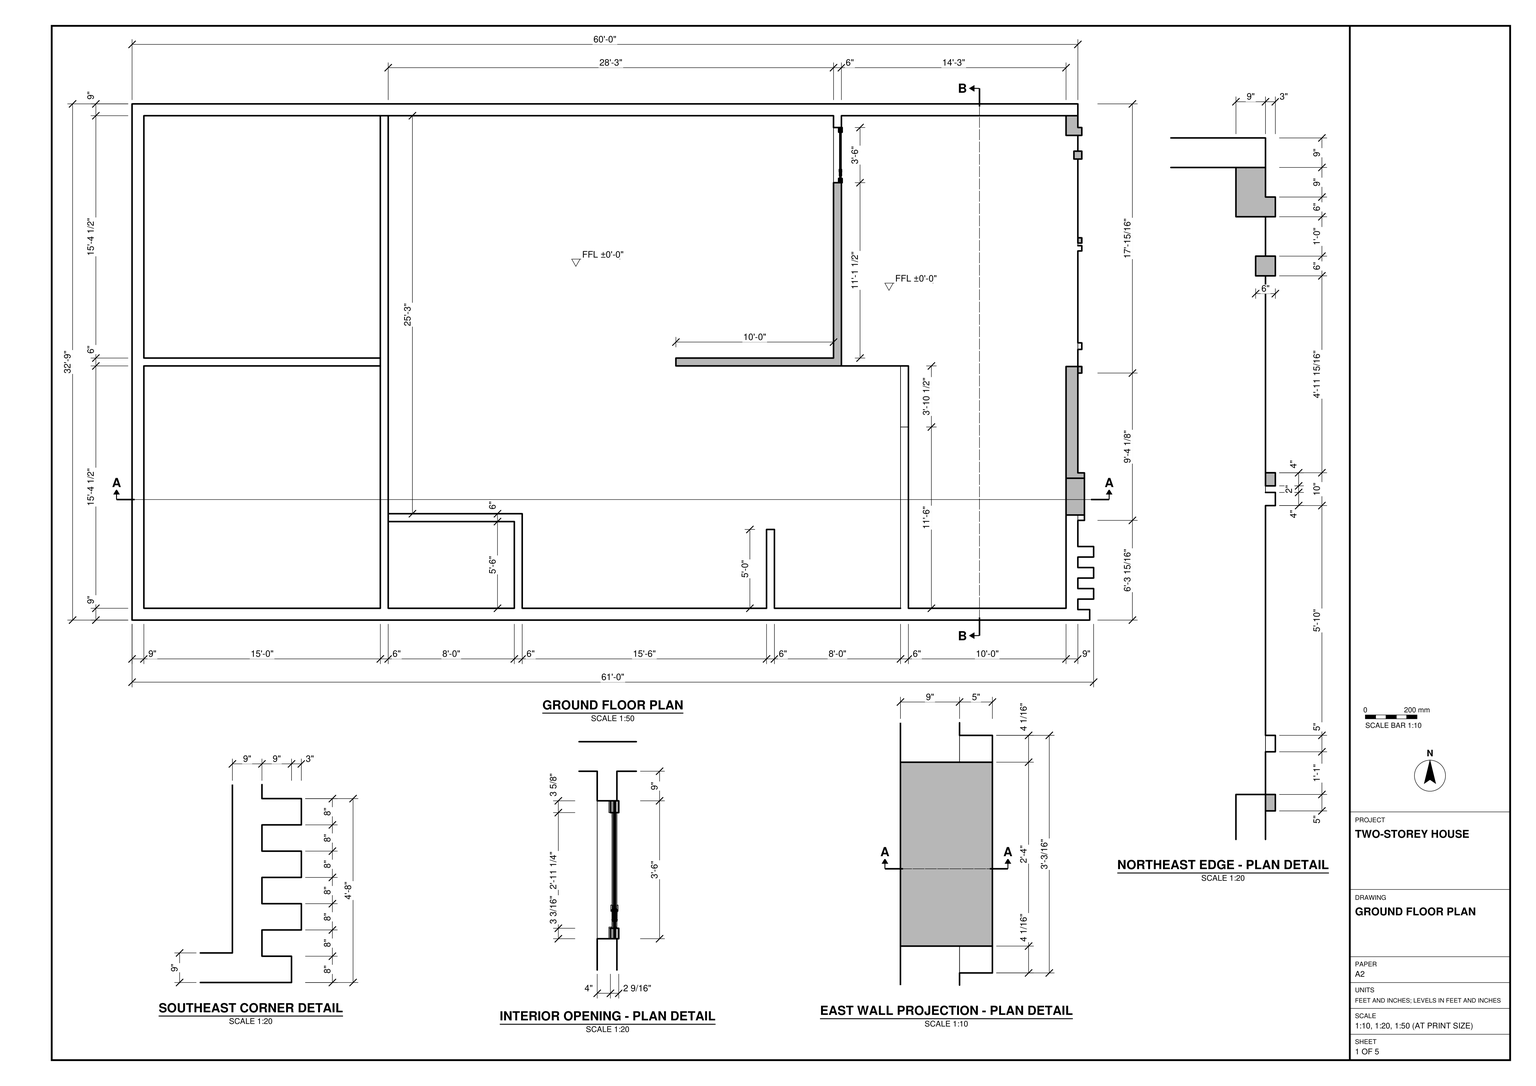
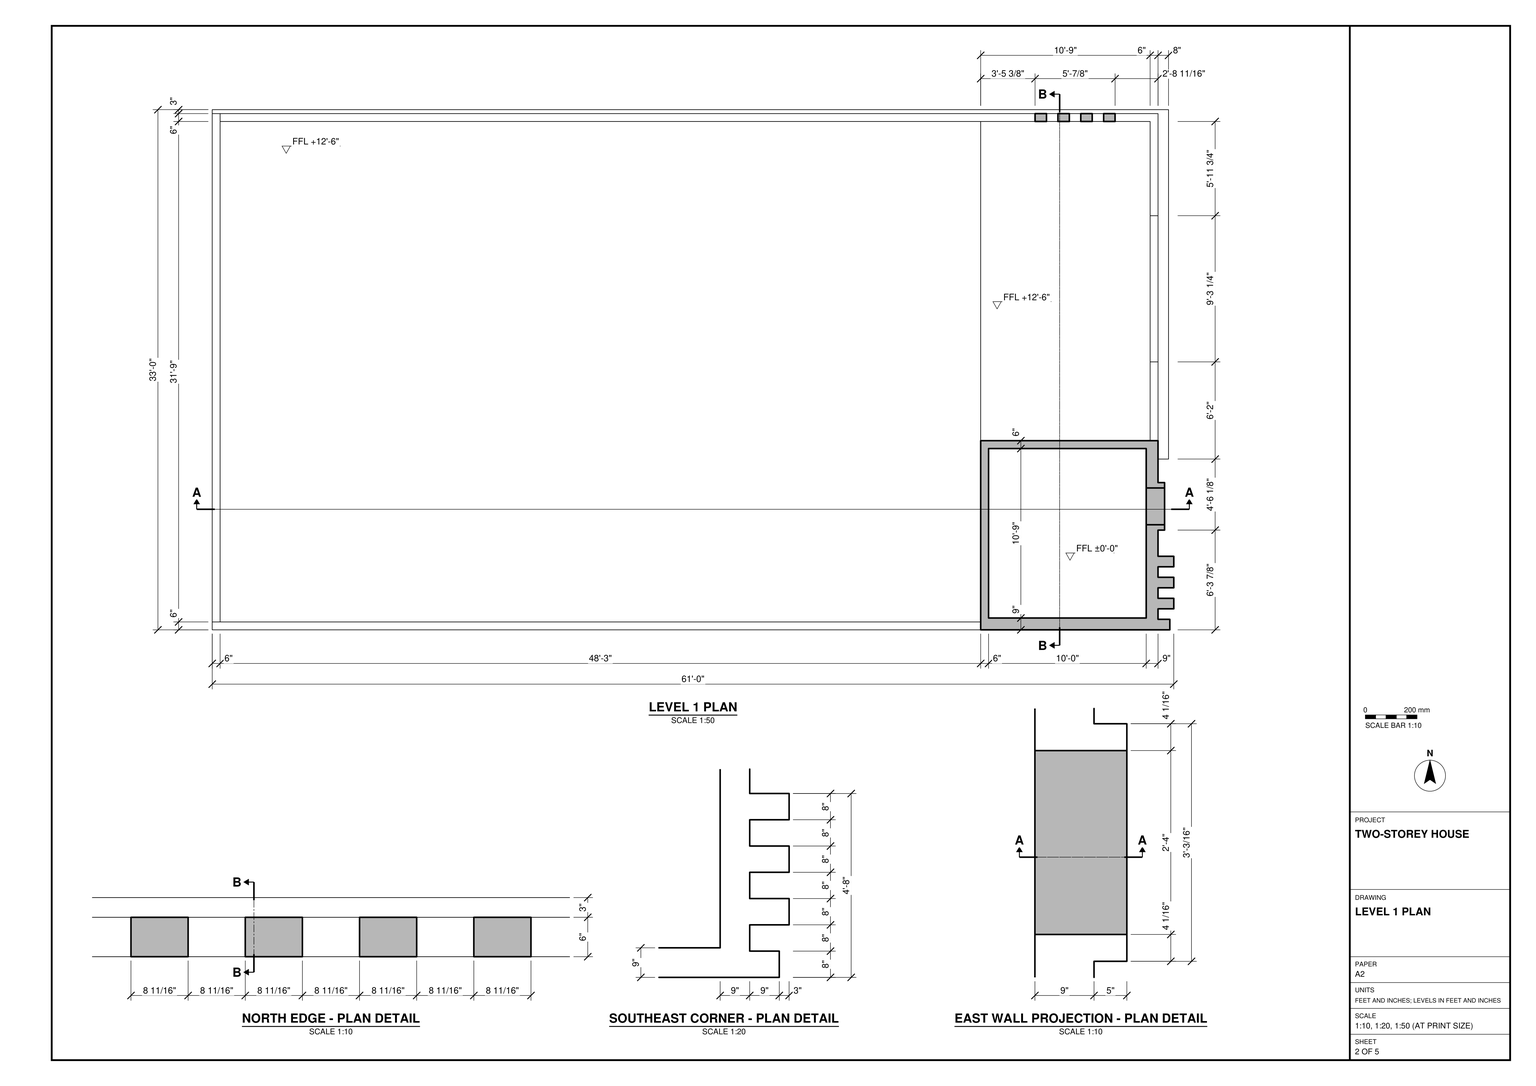
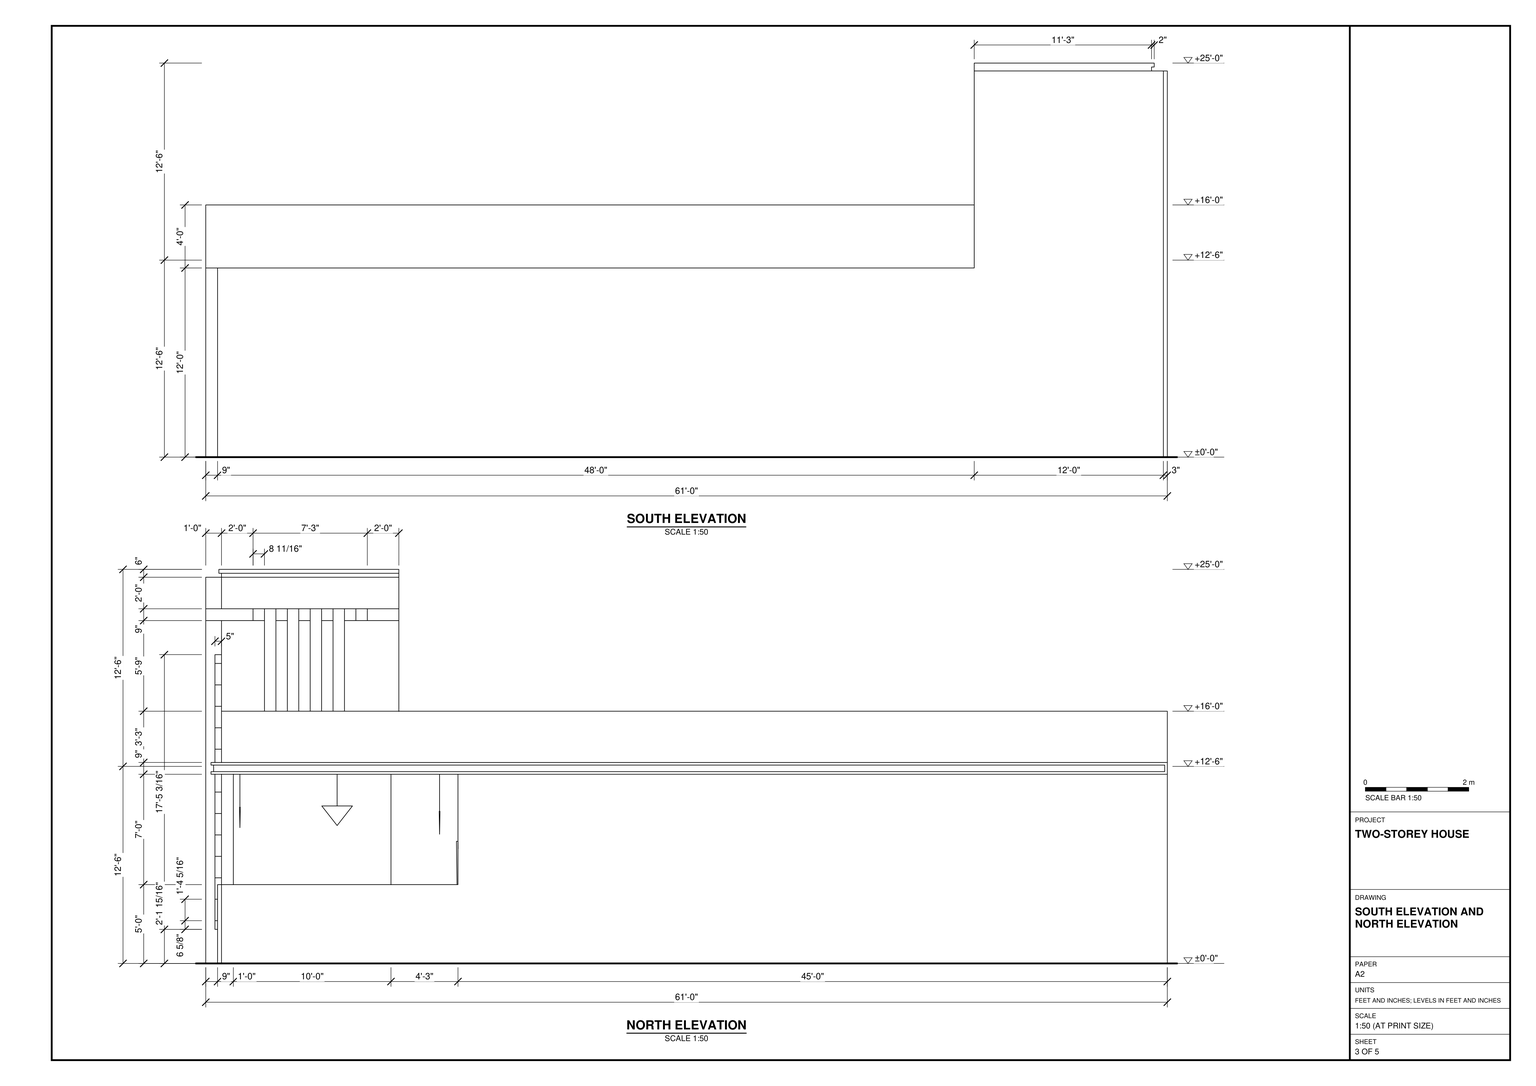
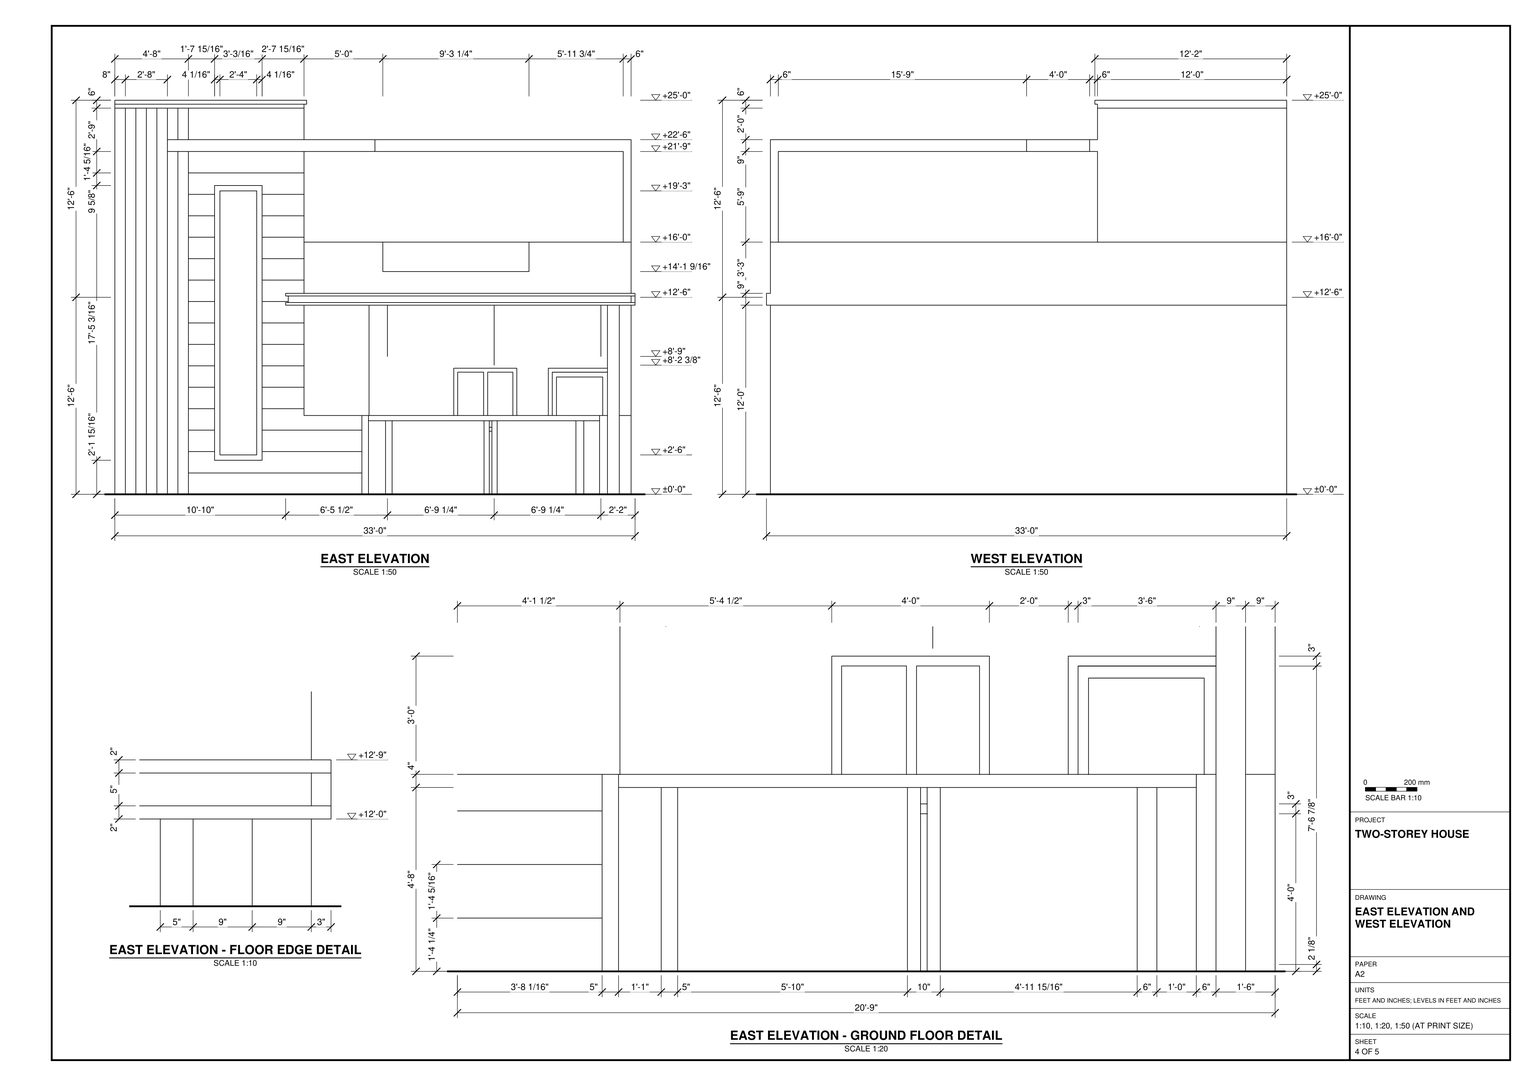
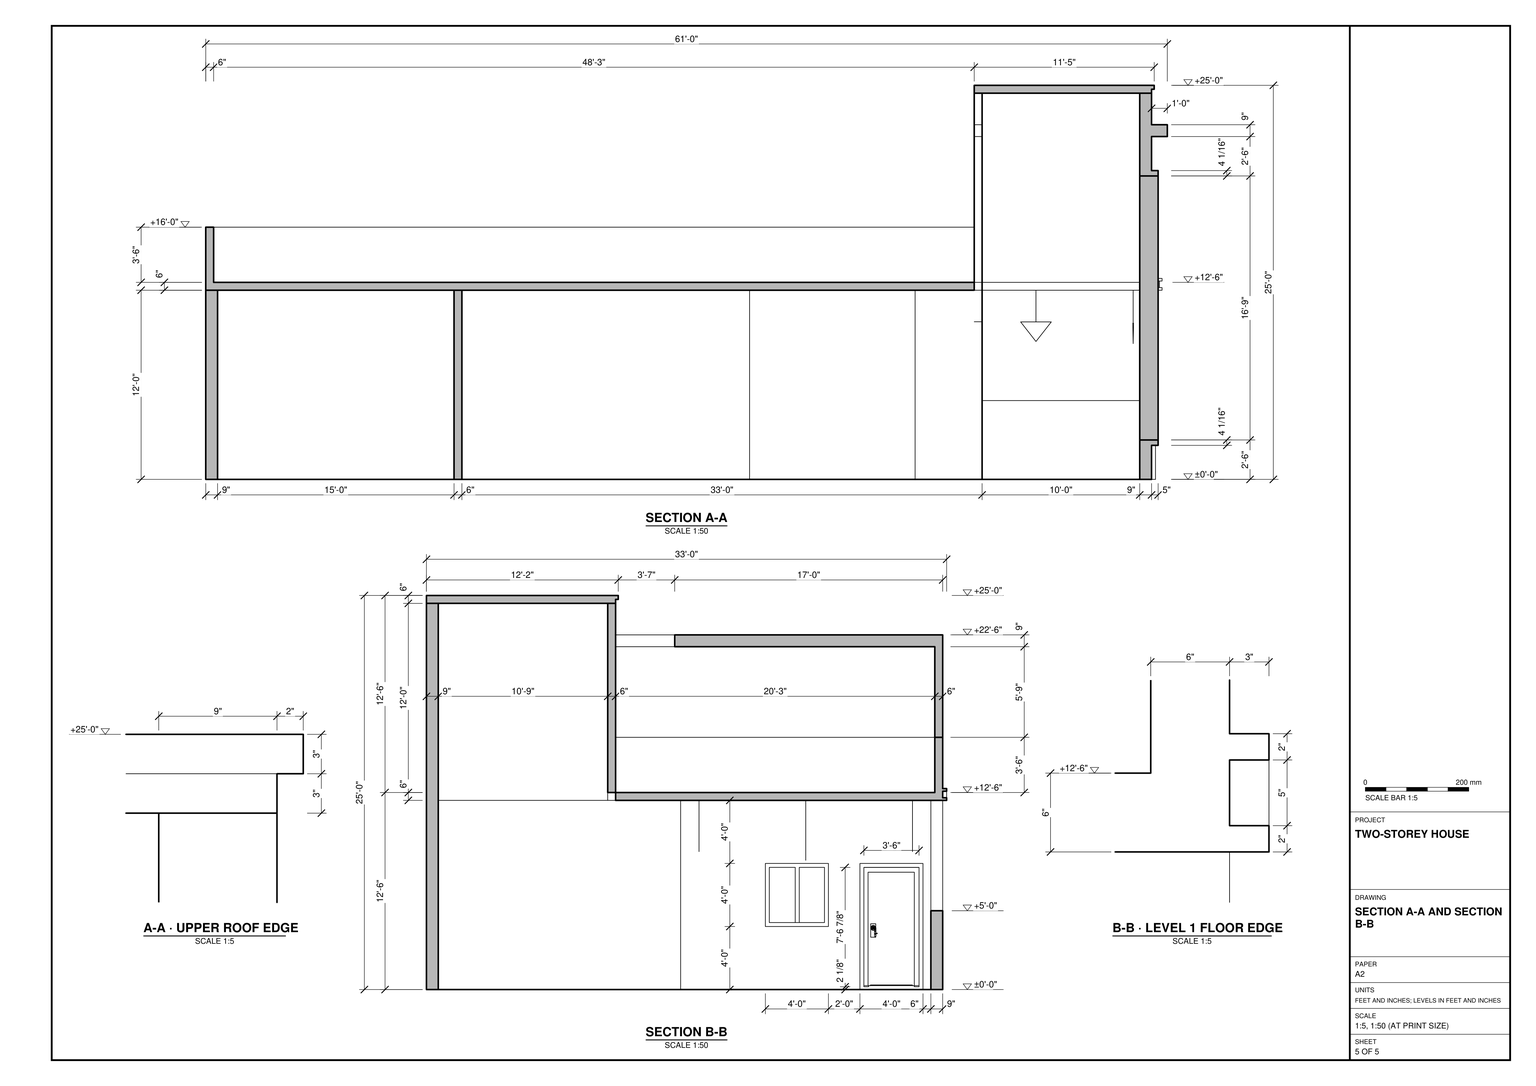
Build the two-storey house in SketchUp from task_files/diagram_01.pdf. Work in feet and inches. The house measures 61'-0" east to west, 33'-0" north to south and 25'-0" high, including the projections. Set the ground floor at ±0'-0" and the upper floor at +12'-6".

Lay out the ground floor with the two rooms at the west end, the small enclosure along the south wall and the returning partitions toward the east. Use the wall thicknesses shown in plan, including the 9" exterior walls and 6" partitions. Set the interior door opening out from the enlarged plan detail. Model the floor and roof slabs, keeping the southeast area marked at ground-floor level open through the upper floor. Follow the elevations for the long, low parapet, the higher roof at the east end and the openings below. Use the edge details to shape the east wall projection, the stepped southeast corner and the spaced vertical members on the upper north face.

Keep walls, slabs, roof elements and any furniture or joinery pieces shown in separate groups or components. Use components for repeated parts. Decor and loose items shown may be represented by any suitable library components. Save one SketchUp model as output_files/two_storey_house_with_a_raised_east_end.skp.

# SketchUp Ruby script. Lengths in inches.
U = 1.inch
M = Sketchup.active_model
def pt(a) = Geom::Point3d.new(a.map { |v| v * U })
def face(e, loops, mat)
  f = e.add_face(loops[0].map { |a| pt(a) })
  loops[1..].each { |l| e.add_face(l.map { |a| pt(a) }).erase! }
  f.material = f.back_material = mat if mat
  f
end
# faces: each face lists its corners as indices into pts; further lists are holes
def faces(e, pts, list, mat = nil) = list.each { |f| face(e, (f[0].is_a?(Array) ? f : [f]).map { |l| l.map { |i| pts[i] } }, mat) }
# xy, xz, yz: faces in a plane at the given z, y or x. An outline is a flat list of corners, or four numbers for a rectangle; further outlines are holes
def ring(l) = l.size == 4 ? [[l[0], l[1]], [l[2], l[1]], [l[2], l[3]], [l[0], l[3]]] : l.each_slice(2).to_a
def flat(e, list, mat, &to3) = list.each { |f| face(e, (f[0].is_a?(Array) ? f : [f]).map { |l| ring(l).map { |u, v| to3.(u, v) } }, mat) }
def xy(e, z, list, mat = nil) = flat(e, list, mat) { |x, y| [x, y, z] }
def xz(e, y, list, mat = nil) = flat(e, list, mat) { |x, z| [x, y, z] }
def yz(e, x, list, mat = nil) = flat(e, list, mat) { |y, z| [x, y, z] }
def lines(e, pts, list) = list.each { |a, b| e.add_line(pt(pts[a]), pt(pts[b])) }
# prism: a flat outline (further loops are holes) pulled along v
def prism(e, loops, v, mat = nil)
  f = face(e, loops, mat); d = Geom::Vector3d.new(v.map { |x| x * U })
  f.pushpull(f.normal.samedirection?(d) ? d.length : -d.length)
end
def box(e, o, s, mat = nil) = prism(e, [[o, [o[0] + s[0], o[1], o[2]], [o[0] + s[0], o[1] + s[1], o[2]], [o[0], o[1] + s[1], o[2]]]], [0, 0, s[2]], mat)
def at(x, y, z, deg = 0) = Geom::Transformation.translation(pt([x, y, z])) * Geom::Transformation.rotation(ORIGIN, Z_AXIS, deg.degrees)
def axes(o, x, y, z) = Geom::Transformation.new([*x, 0, *y, 0, *z, 0, *pt(o).to_a, 1])
def part(name) = M.definitions.add(name)
# library, detail: a bought-in or finely detailed component or shape, given as its bounding box
def library(name, o, s) = part(name).tap { |d| box(d.entities, o, s) }
def detail(e, o, s) = box(e.add_group.entities, o, s)
def put(e, d, t, mat = nil) = e.add_instance(d, t).tap { |i| i.material = mat if mat }
def group(e, t, mat = nil) = e.add_group.tap { |g| g.transformation = t; g.material = mat if mat }.entities
root = M.entities
M.materials.add("Glass_Basic_01").color = [161, 173, 186]
M.materials["Glass_Basic_01"].alpha = 0.25
M.materials.add("Glass_Sky Reflection_01").color = [126, 138, 183]
M.materials["Glass_Sky Reflection_01"].alpha = 0.25
M.materials.add("M08_Obsidian_Black").color = [30, 30, 30]
M.materials.add("Plywood_01_1K").color = [168, 129, 86]
M.materials.add("ThomThom - Beard1").color = [255, 241, 235]
M.materials.add("ThomThom - Beard2").color = [186, 155, 124]
M.materials.add("ThomThom - Buttons1").color = [92, 94, 102]
M.materials.add("ThomThom - Complexion1").color = [242, 222, 211]
M.materials.add("ThomThom - Hair1").color = [125, 114, 96]
M.materials.add("ThomThom - Trousers1").color = [61, 63, 63]
M.materials.add("ThomThom - Waistcoat2").color = [127, 127, 126]
M.materials.add("Wood_Veneer_15_1K").color = [137, 75, 48]
c1 = library("Sphere Light",[-4.05,-4.05,-4.05],[8.1,8.1,8.1])
c2 = library("Sphere Light\#1",[-3.99,-3.99,-3.99],[7.98,7.98,7.98])
c3 = library("Sphere Light\#2",[-3.78,-3.78,-3.78],[7.56,7.56,7.56])
c4 = library("Sphere Light\#3",[-4.24,-4.24,-4.24],[8.48,8.48,8.48])
c5 = part("Group45\#1")
p = [[0,0,0],[0,0,-6.56],[-1.28,0,-6.56],[8.32,-12.92,0],[-8.32,-12.92,0],[8.32,12.92,0],
  [8.32,0,0],[-8.32,12.92,0],[1.28,0,-6.56],[-8.32,0,0],[0,0,-10.62]]
lines(c5.entities,p,[[0,1],[1,2],[3,4],[5,6],[7,5],[1,8],[9,0],[0,6],[8,10],[4,9],[6,3],[2,10],
  [9,7]])
c6 = part("Rectangle Light\#4")
put(c6.entities,c5,at(0,0,0))
c7 = part("Group4\#1")
p = [[0,0,0],[0,0,-24.09],[-11.67,0,-24.09],[76,-2,0],[-76,-2,0],[76,2,0],
  [76,0,0],[-76,2,0],[11.67,0,-24.09],[-76,0,0],[0,0,-39]]
lines(c7.entities,p,[[0,1],[1,2],[3,4],[5,6],[7,5],[1,8],[9,0],[0,6],[8,10],[4,9],[6,3],[2,10],
  [9,7]])
c8 = part("Rectangle Light")
put(c8.entities,c7,at(0,0,0))
c9 = part("Group6\#1")
p = [[0,0,0],[0,0,-25.1],[-0.31,0,-25.1],[2,-79.25,0],[-2,-79.25,0],[2,79.25,0],
  [2,0,0],[-2,79.25,0],[0.31,0,-25.1],[-2,0,0],[0,0,-40.625]]
lines(c9.entities,p,[[0,1],[1,2],[3,4],[5,6],[7,5],[1,8],[9,0],[0,6],[8,10],[4,9],[6,3],[2,10],
  [9,7]])
c10 = part("Rectangle Light\#1")
put(c10.entities,c9,at(0,0,0))
c11 = part("Group8\#1")
p = [[0,0,0],[0,0,-24.09],[-11.67,0,-24.09],[76,-2,0],[-76,-2,0],[76,2,0],
  [76,0,0],[-76,2,0],[11.67,0,-24.09],[-76,0,0],[0,0,-39]]
lines(c11.entities,p,[[0,1],[1,2],[3,4],[5,6],[7,5],[1,8],[9,0],[0,6],[8,10],[4,9],[6,3],[2,10],
  [9,7]])
c12 = part("Rectangle Light\#2")
put(c12.entities,c11,at(0,0,0))
c13 = part("Group10\#1")
p = [[0,0,0],[0,0,-28.1875],[-0.31,0,-28.1875],[2,-89.25,0],[-2,-89.25,0],[2,89.25,0],
  [2,0,0],[-2,89.25,0],[0.31,0,-28.1875],[-2,0,0],[0,0,-45.625]]
lines(c13.entities,p,[[0,1],[1,2],[3,4],[5,6],[7,5],[1,8],[9,0],[0,6],[8,10],[4,9],[6,3],[2,10],
  [9,7]])
c14 = part("Rectangle Light\#3")
put(c14.entities,c13,at(0,0,0))
c15 = library("porta+4",[0.2,-5.42,1.33],[46.55,4.72,83.21])
box(root,[720,188.07,0],[3,5,60],"ThomThom - Trousers1")
xy(root,294,[[585,0,720,144]])
xy(root,297,[[720,0,722,146],[585,144,720,146]])
xy(root,300,[[585,0,722,146]])
xz(root,0,[[585,294,720,294,720,297,722,297,722,300,585,300]])
xz(root,144,[[585,294,720,297]],"ThomThom - Hair1")
xz(root,146,[[585,297,722,300]],"M08_Obsidian_Black")
yz(root,585,[[0,294,0,300,146,300,146,297,144,297,144,294]])
yz(root,720,[[291.04,0,351,56],[357,0,369,56]],"ThomThom - Beard2")
yz(root,720,[[0,294,144,297]],"ThomThom - Hair1")
yz(root,722,[[0,297,146,300]],"M08_Obsidian_Black")
p = [[540,330,0],[540,378,0],[591,147,144],[591,153,144],[540,199.5,144],[540,199.5,150],
  [585,6,150],[585,0,150],[714,144,150],[720,144,150],[720,206.07,0],[720,206.07,56],
  [720,211.07,0],[720,211.07,56],[720,206.07,60],[720,211.07,60]]
lines(root,p,[[0,1],[2,3],[4,5],[6,7],[8,9],[10,11],[12,10],[13,12],[11,13],[14,15]])
put(root,c1,at(676.54,235.45,147.64))
put(root,c2,at(676.65,341.61,147.64))
put(root,c3,at(583.32,235.52,147.64))
put(root,c4,at(583.32,341.35,147.64))
put(root,c6,axes([521.69,287.86,143.99],[1,0,0],[0,-1,0],[0,0,1]))
g1 = group(root,at(0,0,144))
box(g1,[717,351,-144],[6,6,56],"ThomThom - Trousers1")
xy(g1,-144,[[711,369,711,384,720,384,720,375,723,375,723,369]])
xy(g1,-84,[[711,369,723,375]],"ThomThom - Waistcoat2")
xy(g1,0,[[0,0,0,396,720,396,720,384,540,384,540,193.5,591,193.5,591,144,585,144,585,0],[720,130,728,384],[[552,205.5,708,372],[556,209.5,704,368]],[720,384,728,396]])
xy(g1,0,[[[591,144,591,193.5,540,193.5,540,384,711,384,711,375,720,375,720,144],[552,205.5,708,372]],[[556,209.5,704,368],[583.11,231.55,584.15,231.6875,585.11,232.09,585.94,232.72,586.58,233.55,586.98,234.52,587.11,235.55,586.98,236.59,586.58,237.55,585.94,238.38,585.11,239.02,584.15,239.42,583.11,239.55,582.08,239.42,581.11,239.02,580.28,238.38,579.65,237.55,579.25,236.59,579.11,235.55,579.25,234.52,579.65,233.55,580.28,232.72,581.11,232.09,582.08,231.6875],[676.55,231.55,677.58,231.6875,678.55,232.09,679.38,232.72,680.01,233.55,680.41,234.52,680.55,235.55,680.41,236.59,680.01,237.55,679.38,238.38,678.55,239.02,677.58,239.42,676.55,239.55,675.51,239.42,674.55,239.02,673.72,238.38,673.08,237.55,672.69,236.59,672.55,235.55,672.69,234.52,673.08,233.55,673.72,232.72,674.55,232.09,675.51,231.6875],[583.11,337.48,584.15,337.62,585.11,338.01,585.94,338.65,586.58,339.48,586.98,340.44,587.11,341.48,586.98,342.51,586.58,343.48,585.94,344.31,585.11,344.94,584.15,345.34,583.11,345.48,582.08,345.34,581.11,344.94,580.28,344.31,579.65,343.48,579.25,342.51,579.11,341.48,579.25,340.44,579.65,339.48,580.28,338.65,581.11,338.01,582.08,337.62],[676.55,337.48,677.58,337.62,678.55,338.01,679.38,338.65,680.01,339.48,680.41,340.44,680.55,341.48,680.41,342.51,680.01,343.48,679.38,344.31,678.55,344.94,677.58,345.34,676.55,345.48,675.51,345.34,674.55,344.94,673.72,344.31,673.08,343.48,672.69,342.51,672.55,341.48,672.69,340.44,673.08,339.48,673.72,338.65,674.55,338.01,675.51,337.62]]],"ThomThom - Complexion1")
xy(g1,2,[[726,130,728,130,728,396,2,396,2,393,726,393],[720,130,726,132]])
xy(g1,3.64,[[583.11,231.55,582.08,231.6875,581.11,232.09,580.28,232.72,579.65,233.55,579.25,234.52,579.11,235.55,579.25,236.59,579.65,237.55,580.28,238.38,581.11,239.02,582.08,239.42,583.11,239.55,584.15,239.42,585.11,239.02,585.94,238.38,586.58,237.55,586.98,236.59,587.11,235.55,586.98,234.52,586.58,233.55,585.94,232.72,585.11,232.09,584.15,231.6875],[676.55,231.55,675.51,231.6875,674.55,232.09,673.72,232.72,673.08,233.55,672.69,234.52,672.55,235.55,672.69,236.59,673.08,237.55,673.72,238.38,674.55,239.02,675.51,239.42,676.55,239.55,677.58,239.42,678.55,239.02,679.38,238.38,680.01,237.55,680.41,236.59,680.55,235.55,680.41,234.52,680.01,233.55,679.38,232.72,678.55,232.09,677.58,231.6875],[583.11,337.48,582.08,337.62,581.11,338.01,580.28,338.65,579.65,339.48,579.25,340.44,579.11,341.48,579.25,342.51,579.65,343.48,580.28,344.31,581.11,344.94,582.08,345.34,583.11,345.48,584.15,345.34,585.11,344.94,585.94,344.31,586.58,343.48,586.98,342.51,587.11,341.48,586.98,340.44,586.58,339.48,585.94,338.65,585.11,338.01,584.15,337.62],[676.55,337.48,675.51,337.62,674.55,338.01,673.72,338.65,673.08,339.48,672.69,340.44,672.55,341.48,672.69,342.51,673.08,343.48,673.72,344.31,674.55,344.94,675.51,345.34,676.55,345.48,677.58,345.34,678.55,344.94,679.38,344.31,680.01,343.48,680.41,342.51,680.55,341.48,680.41,340.44,680.01,339.48,679.38,338.65,678.55,338.01,677.58,337.62]])
xy(g1,6,[[6,6,585,387],[585,144,714,387]])
xy(g1,7,[[720,130,726,132],[726,130,728,396],[2,393,720,396],[720,393,726,396]])
xy(g1,9,[[720,130,728,130,728,396,0,396,0,393,720,393]])
xy(g1,25.58,[[714,204,720,315.27]])
xy(g1,48,[[0,0,585,6],[0,6,6,393],[714,144,720,204],[714,315.27,720,315.27,720,393,6,393,6,387,714,387]])
xz(g1,0,[[0,0,585,48]],"Wood_Veneer_15_1K")
xz(g1,6,[[6,6,585,48]])
xz(g1,130,[[720,0,728,2],[720,7,728,9]])
xz(g1,132,[[720,2,726,7]])
xz(g1,144,[[585,0,720,0,720,48,714,48,714,6,585,6]])
xz(g1,204,[[714,25.58,720,48]])
xz(g1,315.27,[[714,25.58,720,48]])
xz(g1,369,[[711,-144,723,-84]],"ThomThom - Waistcoat2")
xz(g1,375,[[720,-144,723,-84]],"ThomThom - Trousers1")
xz(g1,375,[[711,-84,720,0]],"ThomThom - Waistcoat2")
xz(g1,384,[[711,-144,720,0]],"ThomThom - Waistcoat2")
xz(g1,387,[[6,6,714,48]])
xz(g1,393,[[2,2,726,7]],"ThomThom - Buttons1")
xz(g1,393,[[0,9,720,48]],"Wood_Veneer_15_1K")
xz(g1,396,[[0,0,0,9,728,9,728,7,2,7,2,2,728,2,728,0]],"M08_Obsidian_Black")
yz(g1,0,[[0,0,0,48,393,48,393,9,396,9,396,0]],"Wood_Veneer_15_1K")
yz(g1,2,[[393,2,396,7]])
yz(g1,6,[[6,6,387,48]])
yz(g1,585,[[0,0,144,6],[0,6,6,48]])
yz(g1,711,[[369,-144,369,-84,375,-84,375,0,384,0,384,-144]])
yz(g1,714,[[144,6,144,48,204,48,204,25.58,315.27,25.58,315.27,48,387,48,387,6]])
yz(g1,720,[[130,0,130,2,132,2,132,7,130,7,130,9,144,9,144,0]])
yz(g1,720,[[204,25.58,315.27,48]],"Glass_Basic_01")
yz(g1,720,[[375,-144,384,0]],"ThomThom - Waistcoat2")
yz(g1,720,[[144,9,393,9,393,48,315.27,48,315.27,25.58,204,25.58,204,48,144,48]],"Wood_Veneer_15_1K")
yz(g1,723,[[369,-144,375,-84]],"ThomThom - Trousers1")
yz(g1,726,[[132,2,393,7]],"ThomThom - Buttons1")
yz(g1,728,[[130,0,396,2],[130,7,396,9]],"M08_Obsidian_Black")
p = [[583.11,231.55,0],[582.08,231.6875,0],[582.08,231.6875,3.64],[583.11,231.55,3.64],[584.15,231.6875,0],[584.15,231.6875,3.64],
  [676.55,231.55,0],[675.51,231.6875,0],[675.51,231.6875,3.64],[676.55,231.55,3.64],[677.58,231.6875,0],[677.58,231.6875,3.64],
  [581.11,232.09,0],[581.11,232.09,3.64],[585.11,232.09,0],[585.11,232.09,3.64],[674.55,232.09,0],[674.55,232.09,3.64],
  [678.55,232.09,0],[678.55,232.09,3.64],[580.28,232.72,0],[580.28,232.72,3.64],[585.94,232.72,0],[585.94,232.72,3.64],
  [673.72,232.72,0],[673.72,232.72,3.64],[679.38,232.72,0],[679.38,232.72,3.64],[579.65,233.55,0],[579.65,233.55,3.64],
  [586.58,233.55,0],[586.58,233.55,3.64],[673.08,233.55,0],[673.08,233.55,3.64],[680.01,233.55,0],[680.01,233.55,3.64],
  [579.25,234.52,0],[579.25,234.52,3.64],[586.98,234.52,0],[586.98,234.52,3.64],[672.69,234.52,0],[672.69,234.52,3.64],
  [680.41,234.52,0],[680.41,234.52,3.64],[579.11,235.55,0],[579.11,235.55,3.64],[587.11,235.55,0],[587.11,235.55,3.64],
  [672.55,235.55,0],[672.55,235.55,3.64],[680.55,235.55,0],[680.55,235.55,3.64],[579.25,236.59,0],[579.25,236.59,3.64],
  [586.98,236.59,0],[586.98,236.59,3.64],[672.69,236.59,0],[672.69,236.59,3.64],[680.41,236.59,0],[680.41,236.59,3.64],
  [579.65,237.55,0],[579.65,237.55,3.64],[586.58,237.55,0],[586.58,237.55,3.64],[673.08,237.55,0],[673.08,237.55,3.64],
  [680.01,237.55,0],[680.01,237.55,3.64],[580.28,238.38,0],[580.28,238.38,3.64],[585.94,238.38,0],[585.94,238.38,3.64],
  [673.72,238.38,0],[673.72,238.38,3.64],[679.38,238.38,0],[679.38,238.38,3.64],[581.11,239.02,0],[581.11,239.02,3.64],
  [585.11,239.02,0],[585.11,239.02,3.64],[674.55,239.02,0],[674.55,239.02,3.64],[678.55,239.02,0],[678.55,239.02,3.64],
  [582.08,239.42,0],[582.08,239.42,3.64],[584.15,239.42,0],[584.15,239.42,3.64],[675.51,239.42,0],[675.51,239.42,3.64],
  [677.58,239.42,0],[677.58,239.42,3.64],[583.11,239.55,0],[583.11,239.55,3.64],[676.55,239.55,0],[676.55,239.55,3.64],
  [583.11,337.48,0],[582.08,337.62,0],[582.08,337.62,3.64],[583.11,337.48,3.64],[584.15,337.62,0],[584.15,337.62,3.64],
  [676.55,337.48,0],[675.51,337.62,0],[675.51,337.62,3.64],[676.55,337.48,3.64],[677.58,337.62,0],[677.58,337.62,3.64],
  [581.11,338.01,0],[581.11,338.01,3.64],[585.11,338.01,0],[585.11,338.01,3.64],[674.55,338.01,0],[674.55,338.01,3.64],
  [678.55,338.01,0],[678.55,338.01,3.64],[580.28,338.65,0],[580.28,338.65,3.64],[585.94,338.65,0],[585.94,338.65,3.64],
  [673.72,338.65,0],[673.72,338.65,3.64],[679.38,338.65,0],[679.38,338.65,3.64],[579.65,339.48,0],[579.65,339.48,3.64],
  [586.58,339.48,0],[586.58,339.48,3.64],[673.08,339.48,0],[673.08,339.48,3.64],[680.01,339.48,0],[680.01,339.48,3.64],
  [579.25,340.44,0],[579.25,340.44,3.64],[586.98,340.44,0],[586.98,340.44,3.64],[672.69,340.44,0],[672.69,340.44,3.64],
  [680.41,340.44,0],[680.41,340.44,3.64],[579.11,341.48,0],[579.11,341.48,3.64],[587.11,341.48,0],[587.11,341.48,3.64],
  [672.55,341.48,0],[672.55,341.48,3.64],[680.55,341.48,0],[680.55,341.48,3.64],[579.25,342.51,0],[579.25,342.51,3.64],
  [586.98,342.51,0],[586.98,342.51,3.64],[672.69,342.51,0],[672.69,342.51,3.64],[680.41,342.51,0],[680.41,342.51,3.64],
  [579.65,343.48,0],[579.65,343.48,3.64],[586.58,343.48,0],[586.58,343.48,3.64],[673.08,343.48,0],[673.08,343.48,3.64],
  [680.01,343.48,0],[680.01,343.48,3.64],[580.28,344.31,0],[580.28,344.31,3.64],[585.94,344.31,0],[585.94,344.31,3.64],
  [673.72,344.31,0],[673.72,344.31,3.64],[679.38,344.31,0],[679.38,344.31,3.64],[581.11,344.94,0],[581.11,344.94,3.64],
  [585.11,344.94,0],[585.11,344.94,3.64],[674.55,344.94,0],[674.55,344.94,3.64],[678.55,344.94,0],[678.55,344.94,3.64],
  [582.08,345.34,0],[582.08,345.34,3.64],[584.15,345.34,0],[584.15,345.34,3.64],[675.51,345.34,0],[675.51,345.34,3.64],
  [677.58,345.34,0],[677.58,345.34,3.64],[583.11,345.48,0],[583.11,345.48,3.64],[676.55,345.48,0],[676.55,345.48,3.64]]
faces(g1,p,[[0,1,2,3],[4,0,3,5],[6,7,8,9],[10,6,9,11],[1,12,13,2],[14,4,5,15],[7,16,17,8],[18,10,11,19],
  [12,20,21,13],[22,14,15,23],[16,24,25,17],[26,18,19,27],[20,28,29,21],[30,22,23,31],[24,32,33,25],[34,26,27,35],
  [28,36,37,29],[38,30,31,39],[32,40,41,33],[42,34,35,43],[36,44,45,37],[46,38,39,47],[40,48,49,41],[50,42,43,51],
  [44,52,53,45],[54,46,47,55],[48,56,57,49],[58,50,51,59],[52,60,61,53],[62,54,55,63],[56,64,65,57],[66,58,59,67],
  [60,68,69,61],[70,62,63,71],[64,72,73,65],[74,66,67,75],[68,76,77,69],[78,70,71,79],[72,80,81,73],[82,74,75,83],
  [76,84,85,77],[86,78,79,87],[80,88,89,81],[90,82,83,91],[84,92,93,85],[92,86,87,93],[88,94,95,89],[94,90,91,95],
  [96,97,98,99],[100,96,99,101],[102,103,104,105],[106,102,105,107],[97,108,109,98],[110,100,101,111],[103,112,113,104],[114,106,107,115],
  [108,116,117,109],[118,110,111,119],[112,120,121,113],[122,114,115,123],[116,124,125,117],[126,118,119,127],[120,128,129,121],[130,122,123,131],
  [124,132,133,125],[134,126,127,135],[128,136,137,129],[138,130,131,139],[132,140,141,133],[142,134,135,143],[136,144,145,137],[146,138,139,147],
  [140,148,149,141],[150,142,143,151],[144,152,153,145],[154,146,147,155],[148,156,157,149],[158,150,151,159],[152,160,161,153],[162,154,155,163],
  [156,164,165,157],[166,158,159,167],[160,168,169,161],[170,162,163,171],[164,172,173,165],[174,166,167,175],[168,176,177,169],[178,170,171,179],
  [172,180,181,173],[182,174,175,183],[176,184,185,177],[186,178,179,187],[180,188,189,181],[188,182,183,189],[184,190,191,185],[190,186,187,191]])
put(g1,c8,axes([632,207.5,-0.01],[-1,0,0],[0,1,0],[0,0,1]))
put(g1,c10,at(706,288.75,-0.01))
put(g1,c12,at(632,370,-0.01,180))
put(g1,c14,axes([554,288.75,0],[1,0,0],[0,-0.93277,0],[0,0,1.00022]))
g2 = group(root,at(0,-87,0),"ThomThom - Complexion1")
xy(g2,0,[[[0,87,729,87,729,95,720,95,720,103,732,103,732,111,720,111,720,119,732,119,732,127,720,127,720,135,732,135,732,143,720,143,720,280.07,711,280.07,711,96,591,96,591,234,585,234,585,96,489,96,489,156,483,156,483,96,297,96,297,168,195,168,195,471,534,471,534,280.5,540,280.5,540,471,720,471,720,480,0,480],[9,286.5,189,471],[9,96,189,280.5],[195,96,291,162]],[9,96,189,280.5],[195,96,291,162],[297,96,483,96,483,156,489,156,489,96,585,96,585,280.5,414,280.5,414,286.5,534,286.5,534,471,195,471,195,168,297,168],[591,96,711,96,711,280.07,720,280.07,720,293.07,723,293.07,723,298.07,720,298.07,720,368.04,723,368.04,723,372.04,720,372.04,720,374.04,723,374.04,723,378.04,720,378.04,720,471,540,471,540,280.5,591,280.5],
  [414,280.5,534,286.5],[9,286.5,189,471]])
xy(g2,3,[[534,420,540,462]])
xy(g2,25.91,[[720,162.91,725,199.09]])
xy(g2,30,[[711,167,725,195]])
xy(g2,51,[[534,348,540,367.75],[534,367.75,540,370.81],[534,370.81,540,390]])
xy(g2,56,[[711,280.07,720,456.01],[720,293.07,723,298.07],[720,372.04,723,374.04],[720,378.04,723,456.01]])
xy(g2,56,[[720,280.07,723,293.07],[720,298.07,723,368.04],[720,368.04,723,372.04],[720,374.04,723,378.04]],"ThomThom - Trousers1")
xy(g2,60,[[711,231,720,231,720,280.07,723,280.07,723,456.01,711,456.01],[540,471,720,480]])
xy(g2,93,[[534,348,540,367.75],[534,370.81,540,390],[534,420,540,462]])
xy(g2,144,[[[0,87,585,87,585,96,489,96,489,156,483,156,483,96,297,96,297,168,195,168,195,280.5,189,280.5,189,286.5,9,286.5,9,471,534,471,534,286.5,540,286.5,540,480,0,480],[9,96,189,280.5],[195,96,291,162]],[585,231,591,280.5],[189,280.5,195,286.5],[414,280.5,534,286.5],[534,280.5,540,286.5],
  [189,286.5,195,471]])
xy(g2,150,[[591,225,710.33,231],[710.33,225,711,231]])
xy(g2,192,[[626.4,474,635.1,480],[643.8,474,652.5,480],[661.2,474,669.9,480],[678.6,474,687.3,480]])
xy(g2,231,[[711,167,725,195]])
xy(g2,235.09,[[720,162.91,725,199.09]])
xy(g2,261,[[720,127,732,135],[720,143,732,231]])
xy(g2,261,[[585,231,585,285,626.4,285,626.4,474,635.1,474,635.1,285,643.8,285,643.8,474,652.5,474,652.5,285,661.2,285,661.2,474,669.9,474,669.9,285,678.6,285,678.6,474,687.3,474,687.3,285,732,285,732,231,711,231,711,276,594,276,594,231]],"M08_Obsidian_Black")
xy(g2,270,[[720,127,732,135]])
xy(g2,270,[[720,143,732,143,732,285,687.3,285,687.3,480,678.6,480,678.6,285,669.9,285,669.9,480,661.2,480,661.2,285,652.5,285,652.5,480,643.8,480,643.8,285,635.1,285,635.1,480,626.4,480,626.4,285,585,285,585,231,594,231,594,276,711,276,711,231,720,231]],"M08_Obsidian_Black")
xy(g2,294,[[[585,87,729,87,729,95,720,95,720,103,732,103,732,111,720,111,720,119,732,119,732,127,720,127,720,135,732,135,732,143,720,143,720,231,585,231],[591,96,711,225]]])
xz(g2,87,[[0,0,9,144]])
xz(g2,87,[[9,0,729,0,729,294,585,294,585,144,9,144]],"ThomThom - Complexion1")
xz(g2,95,[[720,0,729,294]])
xz(g2,96,[[9,0,189,144],[195,0,291,144],[297,0,483,144],[489,0,585,144],[591,0,711,294]])
xz(g2,103,[[720,0,732,294]])
xz(g2,111,[[720,0,732,294]])
xz(g2,119,[[720,0,732,294]])
xz(g2,127,[[720,0,732,261],[720,270,732,294]])
xz(g2,135,[[720,0,732,261],[720,270,732,294]])
xz(g2,143,[[720,0,732,261],[720,270,732,294]])
xz(g2,156,[[483,0,489,144]])
xz(g2,162,[[195,0,291,144]])
xz(g2,162.91,[[720,25.91,725,32.55],[720,32.55,725,48.87],[720,48.87,725,65.19],[720,65.19,725,81.5],[720,81.5,725,97.82],
  [720,97.82,725,114.14],[720,114.14,725,130.46],[720,130.46,725,146.77],[720,146.77,725,163.09],[720,163.09,725,179.41],
  [720,179.41,725,195.73],[720,195.73,725,212.05],[720,212.05,725,228.36],[720,228.36,725,235.09]])
xz(g2,167,[[711,30,725,231]])
xz(g2,168,[[195,0,297,144]])
xz(g2,195,[[711,30,725,150],[711,150,725,231]])
xz(g2,199.09,[[720,25.91,725,32.55],[720,32.55,725,48.87],[720,48.87,725,65.19],[720,65.19,725,81.5],[720,81.5,725,97.82],
  [720,97.82,725,114.14],[720,114.14,725,130.46],[720,130.46,725,146.77],[720,146.77,725,150],[720,150,725,163.09],
  [720,163.09,725,179.41],[720,179.41,725,195.73],[720,195.73,725,212.05],[720,212.05,725,228.36],[720,228.36,725,235.09]])
xz(g2,225,[[591,150,711,294]])
xz(g2,231,[[711,60,720,150],[585,144,591,150],[591,261,594,270]])
xz(g2,231,[[585,150,585,261,594,261,594,270,585,270,585,294,720,294,720,270,711,270,711,261,720,261,720,150]],"ThomThom - Complexion1")
xz(g2,276,[[594,261,711,270]],"ThomThom - Buttons1")
xz(g2,280.07,[[711,0,720,56]])
xz(g2,280.07,[[720,56,723,60]],"ThomThom - Trousers1")
xz(g2,280.5,[[9,0,189,144],[414,0,540,144]])
xz(g2,280.5,[[540,0,591,144]],"ThomThom - Beard1")
xz(g2,285,[[585,261,609,270],[609,261,617.7,270],[617.7,261,626.4,270],[635.1,261,643.8,270],[652.5,261,661.2,270],
  [669.9,261,678.6,270],[687.3,261,696,270],[696,261,732,270]],"ThomThom - Waistcoat2")
xz(g2,286.5,[[9,0,189,144],[414,0,534,144]])
xz(g2,293.07,[[720,0,723,56]],"ThomThom - Trousers1")
xz(g2,298.07,[[720,0,723,56]],"ThomThom - Trousers1")
xz(g2,348,[[534,51,540,93]])
xz(g2,367.75,[[534,51,540,93]])
xz(g2,368.04,[[720,0,723,56]],"ThomThom - Trousers1")
xz(g2,370.81,[[534,51,540,93]])
xz(g2,372.04,[[720,0,723,56]],"ThomThom - Trousers1")
xz(g2,374.04,[[720,0,723,56]],"ThomThom - Trousers1")
xz(g2,378.04,[[720,0,723,56]],"ThomThom - Trousers1")
xz(g2,390,[[534,51,540,93]])
xz(g2,420,[[534,3,540,93]])
xz(g2,456.01,[[711,56,723,60]])
xz(g2,462,[[534,3,540,93]])
xz(g2,471,[[9,0,189,144],[189,0,195,144],[195,0,534,144],[540,0,720,60]])
xz(g2,474,[[626.4,192,635.1,261],[643.8,192,652.5,261],[661.2,192,669.9,261],[678.6,192,687.3,261]],"M08_Obsidian_Black")
xz(g2,480,[[626.4,192,635.1,270],[643.8,192,652.5,270],[661.2,192,669.9,270],[678.6,192,687.3,270]],"M08_Obsidian_Black")
xz(g2,480,[[0,0,0,144,540,144,540,60,720,60,720,0]],"ThomThom - Beard1")
yz(g2,0,[[87,0,480,144]],"ThomThom - Complexion1")
yz(g2,9,[[96,0,280.5,144],[286.5,0,471,144]])
yz(g2,189,[[96,0,280.5,144],[280.5,0,286.5,144],[286.5,0,471,144]])
yz(g2,195,[[96,0,162,144],[162,0,168,144],[168,0,471,144]])
yz(g2,291,[[96,0,162,144]])
yz(g2,297,[[96,0,168,144]])
yz(g2,414,[[280.5,0,286.5,144]])
yz(g2,483,[[96,0,156,144]])
yz(g2,489,[[96,0,156,144]])
yz(g2,534,[[[286.5,0,471,144],[420,3,462,93],[348,51,367.75,93],[370.81,51,390,93]]])
yz(g2,540,[[471,60,480,144]])
yz(g2,540,[[348,51,367.75,93],[370.81,51,390,93]],"Glass_Basic_01")
yz(g2,540,[[[280.5,0,417,0,417,96,465,96,465,0,471,0,471,144,280.5,144],[345,48,393,96]],[[417,0,465,96],[420,3,462,93]],[[345,48,393,96],[348,51,367.75,93],[370.81,51,390,93]]],"Plywood_01_1K")
yz(g2,585,[[87,144,87,294,231,294,231,270,237,270,237,261,231,261,231,144]],"ThomThom - Complexion1")
yz(g2,585,[[237,261,285,270]],"ThomThom - Waistcoat2")
yz(g2,591,[[96,144,225,294],[225,144,231,150],[225,261,231,270]])
yz(g2,591,[[96,0,280.5,144]],"ThomThom - Beard1")
yz(g2,594,[[231,261,276,270]],"ThomThom - Buttons1")
yz(g2,626.4,[[474,192,474,261,285,261,285,270,480,270,480,192]],"M08_Obsidian_Black")
yz(g2,635.1,[[474,192,480,192,480,270,285,270,285,261,474,261]],"M08_Obsidian_Black")
yz(g2,643.8,[[474,192,474,261,285,261,285,270,480,270,480,192]],"M08_Obsidian_Black")
yz(g2,652.5,[[474,192,480,192,480,270,285,270,285,261,474,261]],"M08_Obsidian_Black")
yz(g2,661.2,[[474,192,474,261,285,261,285,270,480,270,480,192]],"M08_Obsidian_Black")
yz(g2,669.9,[[474,192,480,192,480,270,285,270,285,261,474,261]],"M08_Obsidian_Black")
yz(g2,678.6,[[474,192,474,261,285,261,285,270,480,270,480,192]],"M08_Obsidian_Black")
yz(g2,687.3,[[474,192,480,192,480,270,285,270,285,261,474,261]],"M08_Obsidian_Black")
yz(g2,711,[[225,261,231,270]])
yz(g2,711,[[167,30,195,231]],"Glass_Sky Reflection_01")
yz(g2,711,[[231,261,276,270]],"ThomThom - Buttons1")
yz(g2,711,[[[96,0,96,294,225,294,225,150,231,150,231,60,456.01,60,456.01,56,280.07,56,280.07,0],[167,30,195,231]]],"ThomThom - Waistcoat2")
yz(g2,720,[[471,0,480,60]])
yz(g2,720,[[280.07,0,293.07,56],[298.07,0,368.04,56]],"ThomThom - Beard2")
yz(g2,720,[[374.04,0,378.04,56],[280.07,56,456.01,60]],"ThomThom - Trousers1")
yz(g2,720,[[95,0,103,294],[111,0,119,294],[127,0,135,261],[143,0,275.07,16.23],[143,16.23,275.07,16.23,275.07,32.55,199.09,32.55,199.09,25.91,162.91,25.91,162.91,32.55,143,32.55],
  [143,32.55,162.91,48.87],[199.09,32.55,275.07,48.87],[143,48.87,162.91,65.19],[199.09,48.87,275.07,48.87,275.07,60,231,60,231,65.19,199.09,65.19],[143,65.19,162.91,81.5],
  [199.09,65.19,231,81.5],[143,81.5,162.91,97.82],[199.09,81.5,231,97.82],[143,97.82,162.91,114.14],[199.09,97.82,231,114.14],
  [143,114.14,162.91,130.46],[199.09,114.14,231,130.46],[143,130.46,162.91,146.77],[199.09,130.46,231,146.77],[143,146.77,162.91,163.09],
  [199.09,146.77,231,163.09],[143,163.09,162.91,179.41],[199.09,163.09,231,179.41],[143,179.41,162.91,195.73],[199.09,179.41,231,195.73],
  [143,195.73,162.91,212.05],[199.09,195.73,231,212.05],[143,212.05,162.91,228.36],[199.09,212.05,231,228.36],[143,228.36,162.91,228.36,162.91,235.09,199.09,235.09,199.09,228.36,231,228.36,231,244.68,143,244.68],
  [143,244.68,231,261],[127,270,135,294],[143,270,231,294]],"ThomThom - Waistcoat2")
yz(g2,723,[[293.07,0,298.07,56],[368.04,0,372.04,56],[374.04,0,378.04,56],[280.07,56,456.01,60]],"ThomThom - Trousers1")
yz(g2,725,[[167,30,195,231]],"Glass_Sky Reflection_01")
yz(g2,725,[[[162.91,25.91,199.09,235.09],[167,30,195,231]]],"ThomThom - Buttons1")
yz(g2,729,[[87,0,95,294]],"ThomThom - Buttons1")
yz(g2,732,[[103,0,111,294],[119,0,127,294],[135,0,143,261],[135,270,143,294]],"ThomThom - Buttons1")
yz(g2,732,[[127,261,285,270]],"ThomThom - Waistcoat2")
p = [[591,234,120],[585,234,120],[594,231,261],[594,225,261],[585,93,192],[585,93,150],
  [585,231,150],[720,143,-0.09],[720,231,-0.09]]
lines(g2,p,[[0,1],[2,3],[4,5],[5,6],[7,8]])
put(g2,c15,axes([535.72,419.82,0.63],[0,0.90228,0],[-1,0,0],[0,0,1.09264]))
